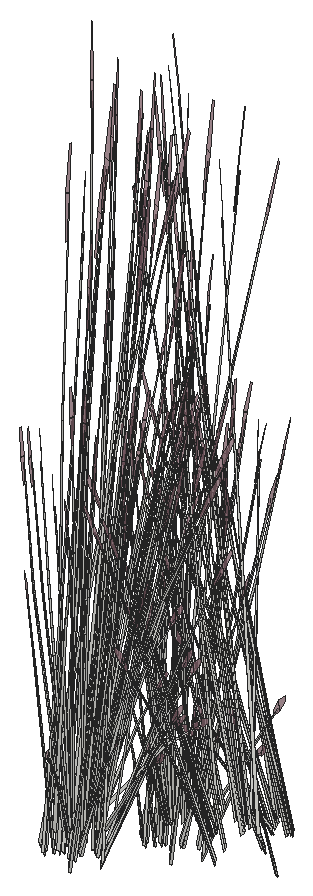
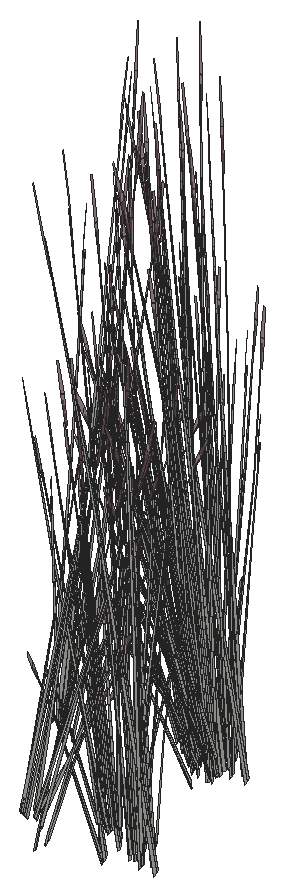
# SketchUp Ruby script. Lengths in inches.
U = 1.inch
M = Sketchup.active_model
def pt(a) = Geom::Point3d.new(a.map { |v| v * U })
def face(e, loops, mat)
  f = e.add_face(loops[0].map { |a| pt(a) })
  loops[1..].each { |l| e.add_face(l.map { |a| pt(a) }).erase! }
  f.material = f.back_material = mat if mat
  f
end
# faces: each face lists its corners as indices into pts; further lists are holes
def faces(e, pts, list, mat = nil) = list.each { |f| face(e, (f[0].is_a?(Array) ? f : [f]).map { |l| l.map { |i| pts[i] } }, mat) }
# xy, xz, yz: faces in a plane at the given z, y or x. An outline is a flat list of corners, or four numbers for a rectangle; further outlines are holes
def ring(l) = l.size == 4 ? [[l[0], l[1]], [l[2], l[1]], [l[2], l[3]], [l[0], l[3]]] : l.each_slice(2).to_a
def flat(e, list, mat, &to3) = list.each { |f| face(e, (f[0].is_a?(Array) ? f : [f]).map { |l| ring(l).map { |u, v| to3.(u, v) } }, mat) }
def xy(e, z, list, mat = nil) = flat(e, list, mat) { |x, y| [x, y, z] }
def xz(e, y, list, mat = nil) = flat(e, list, mat) { |x, z| [x, y, z] }
def yz(e, x, list, mat = nil) = flat(e, list, mat) { |y, z| [x, y, z] }
def lines(e, pts, list) = list.each { |a, b| e.add_line(pt(pts[a]), pt(pts[b])) }
# prism: a flat outline (further loops are holes) pulled along v
def prism(e, loops, v, mat = nil)
  f = face(e, loops, mat); d = Geom::Vector3d.new(v.map { |x| x * U })
  f.pushpull(f.normal.samedirection?(d) ? d.length : -d.length)
end
def box(e, o, s, mat = nil) = prism(e, [[o, [o[0] + s[0], o[1], o[2]], [o[0] + s[0], o[1] + s[1], o[2]], [o[0], o[1] + s[1], o[2]]]], [0, 0, s[2]], mat)
def at(x, y, z, deg = 0) = Geom::Transformation.translation(pt([x, y, z])) * Geom::Transformation.rotation(ORIGIN, Z_AXIS, deg.degrees)
def axes(o, x, y, z) = Geom::Transformation.new([*x, 0, *y, 0, *z, 0, *pt(o).to_a, 1])
def part(name) = M.definitions.add(name)
# library, detail: a bought-in or finely detailed component or shape, given as its bounding box
def library(name, o, s) = part(name).tap { |d| box(d.entities, o, s) }
def detail(e, o, s) = box(e.add_group.entities, o, s)
def put(e, d, t, mat = nil) = e.add_instance(d, t).tap { |i| i.material = mat if mat }
def group(e, t, mat = nil) = e.add_group.tap { |g| g.transformation = t; g.material = mat if mat }.entities
root = M.entities
M.materials.add("LightPink_Translucent").color = [144, 107, 117]
M.materials["LightPink_Translucent"].alpha = 0.75
c1 = part("blade")
p = [[2.15,0.21,22],[0,0.17,0],[0.09,0.45,0],[2.18,0.31,22],[2.29,0.31,22],[0.38,0.45,0],
  [2.48,0.24,33],[2.49,0.24,33],[2.48,0.22,33]]
faces(c1.entities,p,[[0,1,2,3],[4,5,2,3],[6,3,4,7],[8,0,3,6]])
c2 = part("seeds")
p = [[0.3,-0.1,1.38],[-0.01,-0.03,1.59],[-0.01,-0.03,0.03],[0.14,-0.07,-0.07],[0.29,-0.03,3],[0.15,0.01,3.11]]
faces(c2.entities,p,[[0,1,2,3],[1,0,4,5]],"LightPink_Translucent")
c3 = part("blade with seeds")
put(c3.entities,c1,at(0,0,0))
put(c3.entities,c2,axes([2.4,0.25,30.99],[1.5799,-0.05474,1.17369],[-0.12525,1.92788,0.29478],[-0.07173,-0.02425,1.56792]))
put(root,c3,axes([315.15,14.96,47.49],[-0.14352,0.07909,1.26356],[-0.42983,-0.13843,-0.27174],[0.07968,-0.17216,0.54024]))
put(root,c3,axes([315.5,15.54,49.6],[0.01314,-0.36145,-0.62776],[0.55324,0.02428,0.07576],[0.05838,-0.15313,0.88802]))
put(root,c3,axes([316.27,14.98,49.36],[-0.00487,-0.07777,1.54581],[-0.41166,-0.22476,-0.24447],[0.06364,-0.13625,0.12397]))
put(root,c3,axes([314.88,15.36,48.62],[-0.09401,0.13431,1.51428],[-0.3944,-0.27795,0.12244],[0.17792,-0.17323,0.64734]))
put(root,c3,axes([315.39,15.42,49.33],[-0.36145,-0.26255,-0.45151],[0.38183,-0.22994,-0.34973],[0.055,-0.1334,0.86392]))
put(root,c3,axes([315.73,15.32,49.2],[0.34164,-0.20573,-0.31292],[0.3234,0.23491,0.40398],[0.04921,-0.11936,0.77298]))
put(root,c3,axes([316.16,15.2,46.52],[-0.07557,-0.03078,1.55816],[-0.19412,-0.34391,-0.23804],[0.13095,-0.09333,0.26541]))
put(root,c3,axes([315.73,15.4,49.38],[0.35954,0.26661,0.42415],[-0.38183,0.22994,0.34973],[0.06632,-0.12508,0.87768]))
put(root,c3,axes([315.86,15.43,49.375],[0.41493,0.01821,0.05682],[-0.01138,0.27493,0.44729],[0.04342,-0.10531,0.68204]))
put(root,c3,axes([315.55,15.62,49.66],[-0.34164,0.20573,0.31292],[-0.3234,-0.23491,-0.40398],[0.04921,-0.11936,0.77298]))
put(root,c3,axes([316.15,16.17,49.6],[0.26374,-0.30832,-0.62776],[0.46217,0.21911,0.07576],[0.15748,-0.11171,0.88802]))
put(root,c3,axes([316.14,16.03,49.33],[-0.12971,-0.3568,-0.45151],[0.49122,-0.06241,-0.34973],[0.14077,-0.09583,0.86392]))
put(root,c3,axes([316.37,16.28,49.64],[-0.46706,-0.21546,-0.10745],[0.26908,-0.31203,-0.59638],[0.13196,-0.10846,0.90619]))
put(root,c3,axes([313.73,15.21,46.98],[0.47255,-0.19538,-0.43871],[0.28245,0.35034,0],[0.10763,-0.0445,1.3917]))
put(root,c3,axes([316.53,15.89,47.49],[-0.18038,-0.01157,1.26356],[-0.18479,-0.31048,-0.27174],[0.22159,-0.08783,0.54024]))
put(root,c3,axes([317.52,16.1875,49.36],[-0.06595,-0.00297,1.56736],[-0.27386,-0.31799,-0.1481],[0.10998,-0.10455,0.27737]))
put(root,c3,axes([314.29,16.01,47.02],[0.34009,-0.2937,-0.55095],[0.42248,0.26632,-0.1446],[0.13628,-0.07327,1.21613]))
put(root,c3,axes([316.74,15.32,47.64],[-0.16818,0.19891,1.01491],[-0.14456,-0.26725,0.74569],[0.1389,-0.06697,0.22354]))
put(root,c3,axes([316.5,16.0625,49.2],[0.43951,-0.05584,-0.31292],[0.11606,0.31924,0.40398],[0.12595,-0.08575,0.77298]))
put(root,c3,axes([313.92,16.35,47.55],[-0.05884,-0.44587,-0.25709],[0.6128,-0.02696,-0.44182],[0.10791,-0.05939,1.41118]))
put(root,c3,axes([316.14,16.25,49.66],[-0.43951,0.05584,0.31292],[-0.11606,-0.31924,-0.40398],[0.12595,-0.08575,0.77298]))
put(root,c3,axes([326.49,15.88,50.29],[0.09858,0.10879,1.26356],[-0.22716,0.29571,-0.27174],[-0.23325,-0.07068,0.54024]))
put(root,c3,axes([313.84,15.37,46.99],[0.47106,0.09668,-0.27372],[-0.11861,0.34048,0.27372],[0.09497,-0.03926,1.22797]))
put(root,c3,axes([316.54,16.2,49.375],[0.34663,0.16434,0.05682],[-0.20181,0.23402,0.44729],[0.11113,-0.07566,0.68204]))
put(root,c3,axes([316.45,16.13,49.38],[0.12522,0.35963,0.42415],[-0.49122,0.06241,0.34973],[0.14477,-0.08458,0.87768]))
put(root,c3,axes([317.77,16.57,49.36],[0.07006,-0.05952,1.54581],[-0.08968,-0.3651,-0.24447],[0.1758,-0.06922,0.12397]))
put(root,c3,axes([324.27,18.51,50.29],[-0.03058,0.12783,1.26356],[-0.44698,0.10701,-0.27174],[-0.10448,-0.16522,0.54024]))
put(root,c3,axes([316.39,17.12,49.64],[-0.25405,-0.35383,-0.10745],[0.45089,-0.17388,-0.59638],[0.19001,-0.04668,0.90619]))
put(root,c3,axes([316.37,16.82,49.33],[0.13679,-0.35544,-0.45151],[0.46898,0.12183,-0.34973],[0.18882,-0.03259,0.86392]))
put(root,c3,axes([315.625,15.37,47.3],[0.31568,-0.39156,0],[0.52815,0.21836,-0.456],[0.12029,0.04973,1.44655]))
put(root,c3,axes([316.87,16.92,46.95],[-0.3252,0.04689,1.25103],[-0.05176,-0.37326,0.07161],[0.22777,-0.0565,0.71188]))
put(root,c3,axes([317.46,16.59,47.19],[-0.31304,-0.24986,-0.05733],[0.34284,-0.22894,-0.25992],[0.09714,-0.01612,0.85731]))
put(root,c3,axes([315.35,15.57,47.39],[-0.47255,-0.19538,0.43871],[0.28245,-0.35034,0],[0.10763,0.0445,1.3917]))
put(root,c3,axes([316.28,16.95,49.6],[0.44368,-0.17257,-0.62776],[0.24726,0.35524,0.07576],[0.21437,-0.04035,0.88802]))
put(root,c3,axes([316.21,17.01,49.66],[-0.41962,-0.10901,0.31292],[0.12239,-0.31802,-0.40398],[0.16894,-0.02916,0.77298]))
put(root,c3,axes([313.34,16.0625,46.6],[-0.49699,0.15644,1.13921],[-0.15819,-0.44887,0.44265],[0.30518,0.00747,1.29573]))
put(root,c3,axes([314.68,16.18,47.51],[0.09741,-0.34873,0.12794],[0.4759,0.06053,-0.36534],[0.08661,0.03581,1.11991]))
put(root,c3,axes([317.22,16.67,46.52],[-0.02639,-0.05932,1.55816],[0.18302,-0.34702,-0.23804],[0.18462,-0.00499,0.26541]))
put(root,c3,axes([314.47,16.27,47.6],[-0.30332,-0.32798,0.39531],[0.45944,-0.23096,-0.19025],[0.09816,0.04058,1.26923]))
put(root,c3,axes([314.63,16.3,47.55],[0.50979,-0.25942,-0.25709],[0.339,0.36656,-0.44182],[0.12578,0.03723,1.41118]))
put(root,c3,axes([316.66,16.98,49.2],[0.41962,0.10901,-0.31292],[-0.12239,0.31802,0.40398],[0.16894,-0.02916,0.77298]))
put(root,c3,axes([315.91,15.61,46.98],[0.47255,0.19538,-0.43871],[-0.28245,0.35034,0],[0.10763,0.0445,1.3917]))
put(root,c3,axes([315.02,16.72,47.15],[0.56491,0,0],[0,0.40454,0],[0,0,1.5764]))
put(root,c3,axes([315.51,16.59,48.62],[-0.20943,0.00885,1.51428],[0.13893,-0.38357,0.12244],[0.29846,0.02372,0.64734]))
put(root,c3,axes([315.78,15.75,46.99],[0.11861,0.34048,-0.27372],[-0.47106,0.09668,0.27372],[0.09497,0.03926,1.22797]))
put(root,c3,axes([323.91,18.72,49.32],[-0.04891,0.05148,1.55816],[-0.49427,0.11098,-0.23804],[-0.1194,-0.10096,0.26541]))
put(root,c3,axes([316.59,17.11,49.375],[0.18545,0.26643,0.05682],[-0.33817,0.13041,0.44729],[0.14907,-0.02573,0.68204]))
put(root,c3,axes([316.56,17.02,49.38],[-0.14265,0.35629,0.42415],[-0.46898,-0.12183,0.34973],[0.18443,-0.02141,0.87768]))
put(root,c3,axes([314.94,17.62,47.125],[0.53009,-0.13258,-0.16963],[0.18627,0.38191,0.00007],[0.05851,-0.01465,1.53656]))
put(root,c3,axes([315.23,16.35,47.02],[0.52523,0.06406,-0.55095],[-0.11084,0.39517,-0.1446],[0.15674,0.04788,1.21613]))
put(root,c3,axes([317.55,17.04,47.64],[-0.31197,0.06451,1.01491],[0.14684,-0.26661,0.74569],[0.1655,0.01824,0.22354]))
put(root,c3,axes([317.4,18.17,49.36],[-0.04566,-0.03421,1.56736],[0.09987,-0.36669,-0.1481],[0.17984,-0.02343,0.27737]))
put(root,c3,axes([314.95,16.48,47.15],[0.30332,0.32798,-0.39531],[-0.45944,0.23096,0.19025],[0.09816,0.04058,1.26923]))
put(root,c3,axes([317,17.87,48.67],[-0.09664,-0.32847,-0.03085],[0.45676,-0.07551,-0.13989],[0.09538,0.02082,0.4614]))
put(root,c3,axes([315.82,17.86,49.64],[0.02704,-0.39739,-0.10745],[0.51189,0.01086,-0.59638],[0.19715,0.0276,0.90619]))
put(root,c3,axes([316.29,16.8,47.39],[0,-0.39075,0.43871],[0.56491,0,0],[0,0.089,1.3917]))
put(root,c3,axes([315.21,16.68,47.51],[0.47043,-0.11396,0.12794],[0.16474,0.32541,-0.36534],[0,0.07162,1.11991]))
put(root,c3,axes([315.74,17.7,49.66],[-0.28729,-0.24465,0.31292],[0.32804,-0.23159,-0.40398],[0.16667,0.03524,0.77298]))
put(root,c3,axes([316.96,17.47,47.49],[-0.1216,-0.0961,1.26356],[0.15822,-0.31792,-0.27174],[0.24603,0.04307,0.54024]))
put(root,c3,axes([316.27,17.62,49.36],[0.10831,-0.00661,1.54581],[0.29709,-0.30358,-0.24447],[0.19266,0.04007,0.12397]))
put(root,c3,axes([323.6,18.92,49.88],[-0.14565,0.31907,-0.0344],[-0.44829,-0.09815,-0.15595],[-0.06806,-0.05219,0.51438]))
put(root,c3,axes([323.36,20.37,50.1],[-0.63136,0,0],[0,-0.43672,-0.456],[0,-0.09947,1.44655]))
put(root,c3,axes([315.85,17.67,49.6],[0.50473,0.00941,-0.62776],[-0.0339,0.39618,0.07576],[0.21383,0.04181,0.88802]))
put(root,c3,axes([323.47,19.59,50.29],[0.09858,0.10879,1.26356],[-0.22716,0.29571,-0.27174],[-0.23325,-0.07068,0.54024]))
put(root,c3,axes([325.8125,17.47,50.29],[0.17547,0.03208,1.26356],[0.1131,0.32764,-0.27174],[-0.23835,0.06133,0.54024]))
put(root,c3,axes([316.67,16.86,47.3],[0.63136,0,0],[0,0.43672,-0.456],[0,0.09947,1.44655]))
put(root,c3,axes([315.05,16.71,47.55],[0.56863,0.18645,-0.25709],[-0.2738,0.39352,-0.44182],[0.01787,0.09662,1.41118]))
put(root,c3,axes([316.15,17.83,49.2],[0.28729,0.24465,-0.31292],[-0.32804,0.23159,0.40398],[0.16667,0.03524,0.77298]))
put(root,c3,axes([316,17.92,49.375],[-0.02542,0.29714,0.05682],[-0.38391,-0.00815,0.44729],[0.14706,0.03109,0.68204]))
put(root,c3,axes([316.04,17.83,49.38],[-0.3723,0.25748,0.42415],[-0.32109,-0.27343,0.34973],[0.17467,0.04749,0.87768]))
put(root,c3,axes([314.85,18.125,49.66],[-0.07798,-0.31474,0.31292],[0.44579,-0.08311,-0.40398],[0.11974,0.09019,0.77298]))
put(root,c3,axes([316.53,17.16,46.98],[0,0.39075,-0.43871],[-0.56491,0,0],[0,0.089,1.3917]))
put(root,c3,axes([315.12,17.2,48.62],[-0.18755,-0.06732,1.51428],[0.38813,-0.28243,0.12244],[0.24191,0.12741,0.64734]))
put(root,c3,axes([315.15,16.32,49.15],[-0.4363,-0.20303,1.22187],[0.46069,-0.31611,0.5272],[0.14077,0.1905,1.18105]))
put(root,c3,axes([315.8125,17.97,47.64],[-0.28429,-0.11236,1.01491],[0.36709,-0.11416,0.74569],[0.09901,0.0967,0.22354]))
put(root,c3,axes([314.8125,18.29,49.64],[0.30087,-0.33447,-0.10745],[0.43572,0.19269,-0.59638],[0.15146,0.0945,0.90619]))
put(root,c3,axes([314.42,18.57,49.36],[0.00149,-0.04731,1.56736],[0.4327,-0.20872,-0.1481],[0.1503,0.0745,0.27737]))
put(root,c3,axes([315.89,18.39,46.52],[0.03679,-0.05641,1.55816],[0.46313,-0.16615,-0.23804],[0.14041,0.08599,0.26541]))
put(root,c3,axes([324.81,20.88,49.82],[-0.52523,-0.06406,-0.55095],[0.11084,-0.39517,-0.1446],[-0.15674,-0.04788,1.21613]))
put(root,c3,axes([315.28,17.1,47.05],[0.18514,0.35777,-0.61156],[-0.53331,0.12885,-0.16051],[0.02046,0.12115,1.3499]))
put(root,c3,axes([315.17,18.125,49.33],[0.49824,-0.09289,-0.45151],[0.08716,0.35177,-0.34973],[0.13382,0.10081,0.86392]))
put(root,c3,axes([315.86,18.48,47.55],[-0.32378,-0.01225,0.92831],[0.21383,-0.26028,0.51254],[0.12791,0.09247,0.72818]))
put(root,c3,axes([314.92,18.41,49.375],[-0.22948,0.24822,0.05682],[-0.32679,-0.14452,0.44729],[0.10565,0.07958,0.68204]))
put(root,c3,axes([323.12,20.32,49.32],[0.0128,0.06158,1.55816],[-0.25814,0.3216,-0.23804],[-0.18336,-0.01621,0.26541]))
put(root,c3,axes([324.25,21.48,49.79],[-0.11861,-0.34048,-0.27372],[0.47106,-0.09668,0.27372],[-0.09497,-0.03926,1.22797]))
put(root,c3,axes([315.02,18.34,49.38],[-0.5022,0.08967,0.42415],[-0.08716,-0.35177,0.34973],[0.11811,0.10367,0.87768]))
put(root,c3,axes([314.8,17.85,47.49],[0.00891,-0.12953,1.26356],[0.4258,-0.14469,-0.27174],[0.13144,0.15503,0.54024]))
put(root,c3,axes([324.12,21.63,49.78],[-0.47255,-0.19538,-0.43871],[0.28245,-0.35034,0],[-0.10763,-0.0445,1.3917]))
put(root,c3,axes([325.4,20.9375,50.36],[-0.50979,0.25942,-0.25709],[-0.339,-0.36656,-0.44182],[-0.12578,-0.03723,1.41118]))
put(root,c3,axes([315.7,23.91,44.29],[-0.14352,0.07909,1.26356],[-0.42983,-0.13843,-0.27174],[0.07968,-0.17216,0.54024]))
put(root,c3,axes([314.34,17.59,48.62],[-0.11542,-0.12546,1.51428],[0.53333,-0.10562,0.12244],[0.12054,0.19696,0.64734]))
put(root,c3,axes([316.05,24.49,46.4],[0.01314,-0.36145,-0.62776],[0.55324,0.02428,0.07576],[0.05838,-0.15313,0.88802]))
put(root,c3,axes([316.82,23.93,46.17],[-0.00487,-0.07777,1.54581],[-0.41166,-0.22476,-0.24447],[0.06364,-0.13625,0.12397]))
put(root,c3,axes([315.43,24.31,45.43],[-0.09401,0.13431,1.51428],[-0.3944,-0.27795,0.12244],[0.17792,-0.17323,0.64734]))
put(root,c3,axes([316.71,23.65,46.16],[-0.05128,0.02985,1.56736],[-0.5024,-0.1007,-0.1481],[-0.01819,-0.13025,0.27737]))
put(root,c3,axes([315.17,23.28,44.44],[0.06477,0.22786,1.01491],[-0.35932,-0.1262,0.74569],[0.03867,-0.11667,0.22354]))
put(root,c3,axes([324.41,21.86,50.1],[-0.31568,0.39156,0],[-0.52815,-0.21836,-0.456],[-0.12029,-0.04973,1.44655]))
put(root,c3,axes([315.9375,24.37,46.14],[-0.36145,-0.26255,-0.45151],[0.38183,-0.22994,-0.34973],[0.055,-0.1334,0.86392]))
put(root,c3,axes([316.31,24.51,46.45],[-0.55492,-0.01936,-0.10745],[0.01517,-0.36657,-0.59638],[0.03855,-0.14118,0.90619]))
put(root,c3,axes([316.28,24.27,46],[0.34164,-0.20573,-0.31292],[0.3234,0.23491,0.40398],[0.04921,-0.11936,0.77298]))
put(root,c3,axes([316.7,24.15,43.32],[-0.07557,-0.03078,1.55816],[-0.19412,-0.34391,-0.23804],[0.13095,-0.09333,0.26541]))
put(root,c3,axes([322.79,21.18,50.29],[0.17547,0.03208,1.26356],[0.1131,0.32764,-0.27174],[-0.23835,0.06133,0.54024]))
put(root,c3,axes([316.27,24.35,46.18],[0.35954,0.26661,0.42415],[-0.38183,0.22994,0.34973],[0.06632,-0.12508,0.87768]))
put(root,c3,axes([316.41,24.38,46.18],[0.41493,0.01821,0.05682],[-0.01138,0.27493,0.44729],[0.04342,-0.10531,0.68204]))
put(root,c3,axes([316.1,24.57,46.46],[-0.34164,0.20573,0.31292],[-0.3234,-0.23491,-0.40398],[0.04921,-0.11936,0.77298]))
put(root,c3,axes([316.7,25.12,46.4],[0.26374,-0.30832,-0.62776],[0.46217,0.21911,0.07576],[0.15748,-0.11171,0.88802]))
put(root,c3,axes([316.6875,24.98,46.14],[-0.12971,-0.3568,-0.45151],[0.49122,-0.06241,-0.34973],[0.14077,-0.09583,0.86392]))
put(root,c3,axes([316.92,25.23,46.45],[-0.46706,-0.21546,-0.10745],[0.26908,-0.31203,-0.59638],[0.13196,-0.10846,0.90619]))
put(root,c3,axes([325.74,21.22,49.82],[-0.34009,0.2937,-0.55095],[-0.42248,-0.26632,-0.1446],[-0.13628,0.07327,1.21613]))
put(root,c3,axes([314.28,24.16,43.78],[0.47255,-0.19538,-0.43871],[0.28245,0.35034,0],[0.10763,-0.0445,1.3917]))
put(root,c3,axes([317.08,24.84,44.29],[-0.18038,-0.01157,1.26356],[-0.18479,-0.31048,-0.27174],[0.22159,-0.08783,0.54024]))
put(root,c3,axes([318.07,25.14,46.16],[-0.06595,-0.00297,1.56736],[-0.27386,-0.31799,-0.1481],[0.10998,-0.10455,0.27737]))
put(root,c3,axes([314.84,24.96,43.82],[0.34009,-0.2937,-0.55095],[0.42248,0.26632,-0.1446],[0.13628,-0.07327,1.21613]))
put(root,c3,axes([317.29,24.27,44.44],[-0.16818,0.19891,1.01491],[-0.14456,-0.26725,0.74569],[0.1389,-0.06697,0.22354]))
put(root,c3,axes([317.05,25.01,46],[0.43951,-0.05584,-0.31292],[0.11606,0.31924,0.40398],[0.12595,-0.08575,0.77298]))
put(root,c3,axes([322.98,22.05,49.32],[0.06773,0.03904,1.55816],[0.11484,0.36171,-0.23804],[-0.15011,0.07713,0.26541]))
put(root,c3,axes([314.47,25.3,44.36],[-0.05884,-0.44587,-0.25709],[0.6128,-0.02696,-0.44182],[0.10791,-0.05939,1.41118]))
put(root,c3,axes([316.69,25.2,46.46],[-0.43951,0.05584,0.31292],[-0.11606,-0.31924,-0.40398],[0.12595,-0.08575,0.77298]))
put(root,c3,axes([314.39,24.32,43.79],[0.47106,0.09668,-0.27372],[-0.11861,0.34048,0.27372],[0.09497,-0.03926,1.22797]))
put(root,c3,axes([317.09,25.15,46.18],[0.34663,0.16434,0.05682],[-0.20181,0.23402,0.44729],[0.11113,-0.07566,0.68204]))
put(root,c3,axes([316.99,25.08,46.18],[0.12522,0.35963,0.42415],[-0.49122,0.06241,0.34973],[0.14477,-0.08458,0.87768]))
put(root,c3,axes([318.32,25.52,46.17],[0.07006,-0.05952,1.54581],[-0.08968,-0.3651,-0.24447],[0.1758,-0.06922,0.12397]))
put(root,c3,axes([321.54,27.55,45.43],[0.11542,0.12546,1.51428],[-0.53333,0.10562,0.12244],[-0.12054,-0.19696,0.64734]))
put(root,c3,axes([322.42,26.72,46.17],[-0.07723,-0.05479,1.54581],[-0.51538,0.03473,-0.24447],[-0.08225,-0.13104,0.12397]))
put(root,c3,axes([322.96,27.65,46.4],[-0.24099,-0.31773,-0.62776],[0.49607,-0.17707,0.07576],[-0.05635,-0.15352,0.88802]))
put(root,c3,axes([321.39,27.22,44.29],[-0.03058,0.12783,1.26356],[-0.44698,0.10701,-0.27174],[-0.10448,-0.16522,0.54024]))
put(root,c3,axes([322.55,26.94,43.32],[-0.08469,0.01408,1.55816],[-0.46834,-0.15847,-0.23804],[0.00786,-0.13218,0.26541]))
put(root,c3,axes([316.9375,26.07,46.45],[-0.25405,-0.35383,-0.10745],[0.45089,-0.17388,-0.59638],[0.19001,-0.04668,0.90619]))
put(root,c3,axes([316.91,25.77,46.14],[0.13679,-0.35544,-0.45151],[0.46898,0.12183,-0.34973],[0.18882,-0.03259,0.86392]))
put(root,c3,axes([316.17,24.32,44.1],[0.31568,-0.39156,0],[0.52815,0.21836,-0.456],[0.12029,0.04973,1.44655]))
put(root,c3,axes([323.01,27.38,46],[0.15222,-0.30049,-0.31292],[0.44409,0.08764,0.40398],[-0.04072,-0.12098,0.77298]))
put(root,c3,axes([317.42,25.87,43.75],[-0.3252,0.04689,1.25103],[-0.05176,-0.37326,0.07161],[0.22777,-0.0565,0.71188]))
put(root,c3,axes([318.01,25.54,44],[-0.31304,-0.24986,-0.05733],[0.34284,-0.22894,-0.25992],[0.09714,-0.01612,0.85731]))
put(root,c3,axes([322.78,27.58,46.14],[-0.49634,-0.09796,-0.45151],[0.17013,-0.33585,-0.34973],[-0.04551,-0.13522,0.86392]))
put(root,c3,axes([315.9,24.53,44.19],[-0.47255,-0.19538,0.43871],[0.28245,-0.35034,0],[0.10763,0.0445,1.3917]))
put(root,c3,axes([316.83,25.9,46.4],[0.44368,-0.17257,-0.62776],[0.24726,0.35524,0.07576],[0.21437,-0.04035,0.88802]))
put(root,c3,axes([321.89,26.54,46.16],[-0.00942,0.04684,1.56736],[-0.46458,0.16998,-0.1481],[-0.13671,-0.08689,0.27737]))
put(root,c3,axes([314.84,25.28,44.09],[-0.41865,0.35461,0.40429],[-0.49737,-0.31303,0.15865],[0.10093,-0.03539,1.40366]))
put(root,c3,axes([321.79,27.375,46.5],[0.56246,-0.10044,0.47505],[0.09762,0.39398,0.3917],[-0.13228,-0.11611,0.983]))
put(root,c3,axes([316.76,25.96,46.46],[-0.41962,-0.10901,0.31292],[0.12239,-0.31802,-0.40398],[0.16894,-0.02916,0.77298]))
put(root,c3,axes([313.89,25.01,43.41],[-0.49699,0.15644,1.13921],[-0.15819,-0.44887,0.44265],[0.30518,0.00747,1.29573]))
put(root,c3,axes([315.22,25.13,44.3125],[0.09741,-0.34873,0.12794],[0.4759,0.06053,-0.36534],[0.08661,0.03581,1.11991]))
put(root,c3,axes([323.83,22.43,50.29],[0.15933,-0.06164,1.26356],[0.39339,0.18587,-0.27174],[-0.11709,0.16083,0.54024]))
put(root,c3,axes([323.21,27.57,46.45],[-0.49409,0.18193,-0.10745],[-0.24281,-0.32289,-0.59638],[-0.06519,-0.13607,0.90619]))
put(root,c3,axes([321.24,27.02,44.44],[0.26338,0.136,1.01491],[-0.38358,0.08175,0.74569],[-0.08207,-0.10452,0.22354]))
put(root,c3,axes([321.875,27.74,46.4],[-0.43054,-0.18887,-0.62776],[0.30598,-0.33097,0.07576],[-0.15599,-0.11277,0.88802]))
put(root,c3,axes([317.77,25.625,43.32],[-0.02639,-0.05932,1.55816],[0.18302,-0.34702,-0.23804],[0.18462,-0.00499,0.26541]))
put(root,c3,axes([321.73,27.49,46],[-0.07798,-0.31474,-0.31292],[0.44579,-0.08311,0.40398],[-0.11974,-0.09019,0.77298]))
